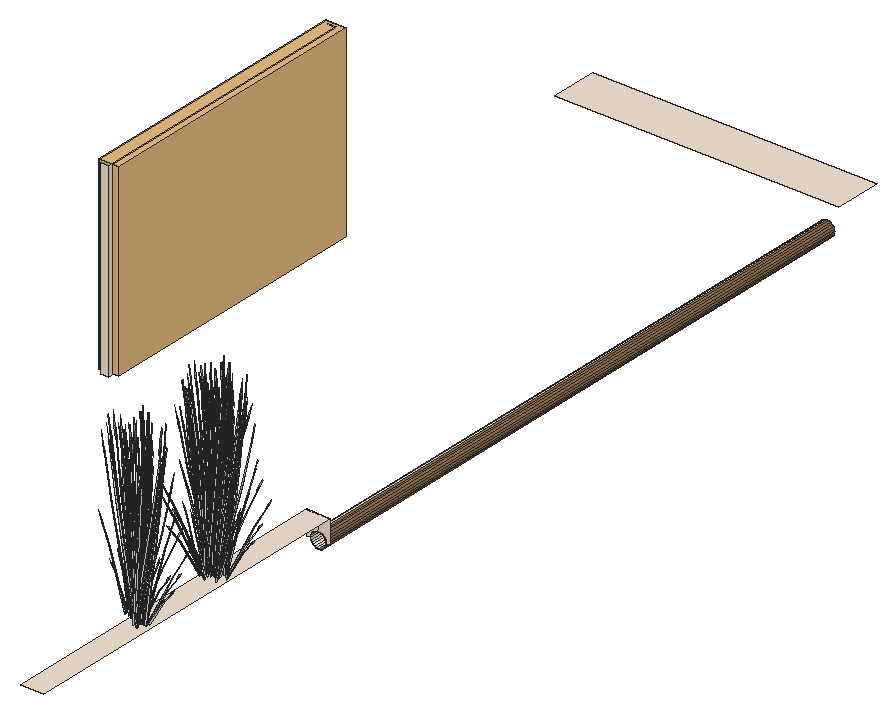
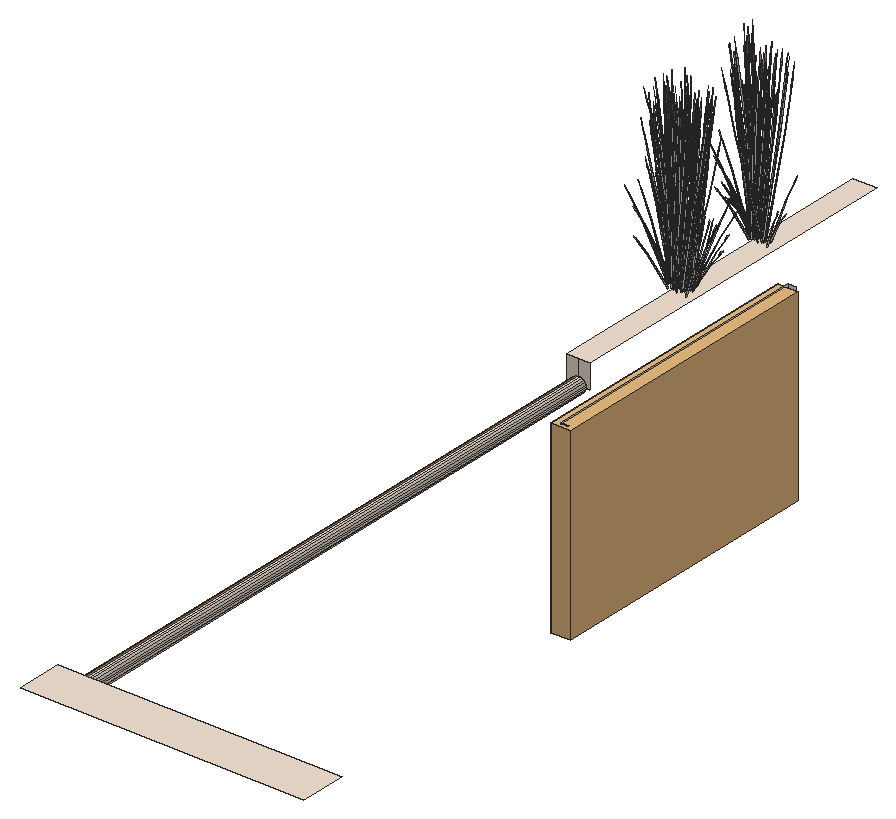
# SketchUp Ruby script. Lengths in inches.
U = 1.inch
M = Sketchup.active_model
def pt(a) = Geom::Point3d.new(a.map { |v| v * U })
def face(e, loops, mat)
  f = e.add_face(loops[0].map { |a| pt(a) })
  loops[1..].each { |l| e.add_face(l.map { |a| pt(a) }).erase! }
  f.material = f.back_material = mat if mat
  f
end
# faces: each face lists its corners as indices into pts; further lists are holes
def faces(e, pts, list, mat = nil) = list.each { |f| face(e, (f[0].is_a?(Array) ? f : [f]).map { |l| l.map { |i| pts[i] } }, mat) }
# xy, xz, yz: faces in a plane at the given z, y or x. An outline is a flat list of corners, or four numbers for a rectangle; further outlines are holes
def ring(l) = l.size == 4 ? [[l[0], l[1]], [l[2], l[1]], [l[2], l[3]], [l[0], l[3]]] : l.each_slice(2).to_a
def flat(e, list, mat, &to3) = list.each { |f| face(e, (f[0].is_a?(Array) ? f : [f]).map { |l| ring(l).map { |u, v| to3.(u, v) } }, mat) }
def xy(e, z, list, mat = nil) = flat(e, list, mat) { |x, y| [x, y, z] }
def xz(e, y, list, mat = nil) = flat(e, list, mat) { |x, z| [x, y, z] }
def yz(e, x, list, mat = nil) = flat(e, list, mat) { |y, z| [x, y, z] }
def lines(e, pts, list) = list.each { |a, b| e.add_line(pt(pts[a]), pt(pts[b])) }
# prism: a flat outline (further loops are holes) pulled along v
def prism(e, loops, v, mat = nil)
  f = face(e, loops, mat); d = Geom::Vector3d.new(v.map { |x| x * U })
  f.pushpull(f.normal.samedirection?(d) ? d.length : -d.length)
end
def box(e, o, s, mat = nil) = prism(e, [[o, [o[0] + s[0], o[1], o[2]], [o[0] + s[0], o[1] + s[1], o[2]], [o[0], o[1] + s[1], o[2]]]], [0, 0, s[2]], mat)
def at(x, y, z, deg = 0) = Geom::Transformation.translation(pt([x, y, z])) * Geom::Transformation.rotation(ORIGIN, Z_AXIS, deg.degrees)
def axes(o, x, y, z) = Geom::Transformation.new([*x, 0, *y, 0, *z, 0, *pt(o).to_a, 1])
def part(name) = M.definitions.add(name)
# library, detail: a bought-in or finely detailed component or shape, given as its bounding box
def library(name, o, s) = part(name).tap { |d| box(d.entities, o, s) }
def detail(e, o, s) = box(e.add_group.entities, o, s)
def put(e, d, t, mat = nil) = e.add_instance(d, t).tap { |i| i.material = mat if mat }
def group(e, t, mat = nil) = e.add_group.tap { |g| g.transformation = t; g.material = mat if mat }.entities
root = M.entities
M.materials.add("C01_Vanilla_Cream").color = [244, 228, 212]
M.materials.add("LightPink_Translucent").color = [144, 107, 117]
M.materials["LightPink_Translucent"].alpha = 0.75
M.materials.add("Wood_Floor_01_1K").color = [146, 111, 76]
c1 = part("blade")
p = [[2.15,0.21,22],[0,0.17,0],[0.09,0.45,0],[2.18,0.31,22],[2.29,0.31,22],[0.38,0.45,0],
  [2.48,0.24,33],[2.49,0.24,33],[2.48,0.22,33]]
faces(c1.entities,p,[[0,1,2,3],[4,5,2,3],[6,3,4,7],[8,0,3,6]])
c2 = part("seeds")
p = [[0.3,-0.1,1.38],[-0.01,-0.03,1.59],[-0.01,-0.03,0.03],[0.14,-0.07,-0.07],[0.29,-0.03,3],[0.15,0.01,3.11]]
faces(c2.entities,p,[[0,1,2,3],[1,0,4,5]],"LightPink_Translucent")
c3 = part("blade with seeds")
put(c3.entities,c1,at(0,0,0))
put(c3.entities,c2,axes([2.4,0.25,30.99],[1.5799,-0.05474,1.17369],[-0.12525,1.92788,0.29478],[-0.07173,-0.02425,1.56792]))
c4 = library("Double casement window",[0,0,0],[5.02,56.42,60])
xy(root,348,[[354,216,360,306.76],[288,324,290,396],[288,468,360,480]],"C01_Vanilla_Cream")
xz(root,306.76,[[354,342,354,348,357,348,357,344,356.48,343.93,356,343.73,355.59,343.41,355.27,343,355.07,342.52,355,342],[359,342,358.93,342.52,358.73,343,358.41,343.41,358,343.73,357.52,343.93,357,344,357,348,360,348,360,342]],"C01_Vanilla_Cream")
xz(root,324,[[288,348,290,396]],"C01_Vanilla_Cream")
xz(root,396,[[288,348,290,396]],"C01_Vanilla_Cream")
yz(root,290,[[[324,348,396,396],[327,351,358.5,393],[361.5,351,393,393]]],"C01_Vanilla_Cream")
p = [[357,306.76,340],[356.48,306.76,340.07],[356.48,468,340.07],[357,468,340],[357.52,306.76,340.07],[357.52,468,340.07],
  [356,306.76,340.27],[356,468,340.27],[358,306.76,340.27],[358,468,340.27],[355.59,306.76,340.59],[355.59,468,340.59],
  [358.41,306.76,340.59],[358.41,468,340.59],[355.27,306.76,341],[355.27,468,341],[358.73,306.76,341],[358.73,468,341],
  [355.07,306.76,341.48],[355.07,468,341.48],[358.93,306.76,341.48],[358.93,468,341.48],[355,306.76,342],[355,468,342],
  [359,306.76,342],[359,468,342],[355.07,306.76,342.52],[355.07,468,342.52],[358.93,306.76,342.52],[358.93,468,342.52],
  [355.27,306.76,343],[355.27,468,343],[358.73,306.76,343],[358.73,468,343],[355.59,306.76,343.41],[355.59,468,343.41],
  [358.41,306.76,343.41],[358.41,468,343.41],[356,306.76,343.73],[356,468,343.73],[358,306.76,343.73],[358,468,343.73],
  [356.48,306.76,343.93],[356.48,468,343.93],[357.52,306.76,343.93],[357.52,468,343.93],[357,306.76,344],[357,468,344]]
faces(root,p,[[0,1,2,3],[1,6,7,2],[6,10,11,7],[10,14,15,11],[14,18,19,15],[18,22,23,19],[22,26,27,23],[26,30,31,27],
  [30,34,35,31],[34,38,39,35],[38,42,43,39],[42,46,47,43]],"C01_Vanilla_Cream")
faces(root,p,[[4,0,3,5],[8,4,5,9],[12,8,9,13],[16,12,13,17],[20,16,17,21],[24,20,21,25],[28,24,25,29],[32,28,29,33],
  [36,32,33,37],[40,36,37,41],[44,40,41,45],[46,44,45,47]],"Wood_Floor_01_1K")
put(root,c3,axes([356.73,248.87,349.86],[0.59825,-0.13076,0.13232],[0.14773,0.48663,0.26315],[-0.05336,-0.0709,1.20305]))
put(root,c3,axes([357.96,247.03,350],[0.56211,-0.32708,-0.21822],[0.3738,0.46216,-0.37502],[0.13869,0.04694,1.19781]))
put(root,c3,axes([355.92,249.08,349.51],[-0.52105,-0.24633,-0.37238],[0.31144,-0.44171,0],[-0.11867,-0.0561,1.18128]))
put(root,c3,axes([359.38,246.16,349.51],[0.52105,0.24633,-0.37238],[-0.31144,0.44171,0],[0.11867,0.0561,1.18128]))
put(root,c3,axes([358.39,247.57,349.65],[0.62289,0,0],[0,0.51004,0],[0,0,1.33805]))
put(root,c3,axes([357.33,248.21,350],[-0.56211,0.32708,-0.21822],[-0.3738,-0.46216,-0.37502],[-0.13869,-0.04694,1.19781]))
put(root,c3,axes([358.57,246.37,349.86],[-0.59825,0.13076,0.13232],[-0.14773,-0.48663,0.26315],[0.05336,0.0709,1.20305]))
put(root,c3,axes([359.23,246.35,349.52],[0.13078,0.42928,-0.23233],[-0.51941,0.1219,0.23233],[0.10471,0.0495,1.0423]))
put(root,c3,axes([358.1875,247.31,349.79],[-0.70367,-0.1038,0.36899],[0.1432,-0.58624,0.1448],[0.10283,0.05661,1.2811]))
put(root,c3,axes([357.625,248.76,349.65],[-0.18165,-0.42474,0],[0.51872,-0.14874,0],[0,0,1.15778]))
put(root,c3,axes([357.28,248.35,349.96],[-0.1074,0.43968,0.1086],[-0.52474,-0.07632,-0.3101],[-0.0955,-0.04515,0.95058]))
put(root,c3,axes([358.31,248.7,349.64],[0.5845,-0.16716,-0.14398],[0.20539,0.48152,0.00006],[0.06452,-0.01848,1.30423]))
put(root,c3,axes([358.51,248.9,349.86],[0.16083,-0.48962,0.13232],[0.58854,0.13856,0.26315],[-0.10167,0.00238,1.20305]))
put(root,c3,axes([358.375,247.79,349.66],[0.38863,0.31822,0],[-0.38863,0.31822,0],[0,0,1.2695]))
put(root,c3,axes([359.43,247.65,349.86],[-0.43742,-0.35886,0.13232],[0.44081,-0.34807,0.26315],[-0.04831,0.07329,1.20305]))
put(root,c3,axes([358.62,247.11,349.54],[0.57914,0.08077,-0.46765],[-0.12221,0.49823,-0.12274],[0.17283,0.06037,1.03225]))
put(root,c3,axes([361.18,247.98,350.07],[-0.34399,0.08133,0.86145],[0.16192,-0.33614,0.63294],[0.18249,0.023,0.18974]))
put(root,c3,axes([357.5,248.95,349.65],[-0.56127,-0.22118,0],[0.27012,-0.45959,0],[0,0,1.2203]))
put(root,c3,axes([357.96,248.36,349.85],[-0.54364,-0.39653,-0.18894],[0.45745,-0.44527,0.41347],[-0.14639,0.04639,1.26162]))
put(root,c3,axes([356.53,249.12,349.86],[0.52105,0.24633,0.37238],[-0.31144,0.44171,0],[-0.11867,-0.0561,1.18128]))
put(root,c3,axes([358.37,247.42,350.04],[0.27012,-0.44393,0.33554],[0.56127,0.21365,-0.16149],[0,0.10233,1.07733]))
put(root,c3,axes([358.27,247.67,349.72],[0,0.56976,-0.04228],[-0.69617,0,0],[0,0.01791,1.34526]))
put(root,c3,axes([358.32,247.27,349.66],[0.33445,0.41351,-0.33554],[-0.50659,0.29119,0.16149],[0.10823,0.05117,1.07733]))
put(root,c3,axes([356.23,249.38,349.78],[-0.34808,0.49367,0],[-0.58235,-0.27531,-0.38706],[-0.13264,-0.0627,1.22783]))
put(root,c3,axes([359.79,247.66,349.86],[0,-0.49266,0.37238],[0.62289,0,0],[0,0.11221,1.18128]))
put(root,c3,axes([358.23,248.03,350.04],[0.60457,-0.03041,0.33554],[0.05467,0.50484,-0.16149],[-0.10823,0.05117,1.07733]))
put(root,c3,axes([358.6,247.52,349.96],[0.51872,-0.14368,0.1086],[0.18165,0.41027,-0.3101],[0,0.09029,0.95058]))
put(root,c3,axes([357.6875,248.28,349.66],[-0.60457,0.03041,-0.33554],[-0.05467,-0.50484,0.16149],[-0.10823,0.05117,1.07733]))
put(root,c3,axes([360.53,248.52,349.94],[-0.13408,-0.12117,1.07251],[0.17446,-0.40083,-0.23066],[0.27128,0.0543,0.45856]))
put(root,c3,axes([358.14,248.96,349.65],[0.56127,0.22118,0],[-0.27012,0.45959,0],[0,0,1.31215]))
put(root,c3,axes([358.36,249.45,349.64],[-0.34375,-0.4954,-0.03857],[0.58235,-0.27531,0.38706],[-0.1435,0.04717,1.22723]))
put(root,c3,axes([358.24,248.25,349.96],[0.41131,0.296,0.1086],[-0.34309,0.33395,-0.3101],[-0.0955,0.04515,0.95058]))
put(root,c3,axes([358.67,249.16,349.86],[0.52105,-0.24633,0.37238],[0.31144,0.44171,0],[-0.11867,0.0561,1.18128]))
put(root,c3,axes([357.93,248.77,349.72],[0.24206,0.56598,-0.04509],[-0.69162,0.19832,0],[0.00845,0.01976,1.2913]))
put(root,c3,axes([358.2,249.38,349.52],[-0.51941,-0.1219,-0.23233],[0.13078,-0.42928,0.23233],[-0.10471,0.0495,1.0423]))
put(root,c3,axes([354.45,248.51,349.94],[0.19348,0.04044,1.07251],[0.1247,0.41309,-0.23066],[-0.26282,0.07733,0.45856]))
put(root,c3,axes([360.21,247.75,349.78],[0.69617,0,0],[0,0.55062,-0.38706],[0,0.12541,1.22783]))
put(root,c3,axes([359.93,248.03,349.65],[-0.69582,-0.00394,-0.03732],[0,-0.55062,0.37457],[-0.02187,0.12535,1.18764]))
put(root,c3,axes([358.43,247.55,350],[0.62699,0.23507,-0.21822],[-0.3019,0.49615,-0.37502],[0.0197,0.12182,1.19781]))
put(root,c3,axes([354.05,249.38,350.07],[0.23202,-0.22328,0.86145],[0.09155,0.35348,0.63294],[-0.16768,0.06329,0.18974]))
put(root,c3,axes([359.79,248.11,349.52],[-0.38863,0.30738,-0.23233],[-0.38863,-0.30738,0.23233],[0,0.09901,1.0423]))
put(root,c3,axes([358.11,248.14,350],[0.06488,0.56215,-0.21822],[-0.6757,0.03399,-0.37502],[-0.11898,0.07488,1.19781]))
put(root,c3,axes([358.36,247.92,349.66],[-0.27012,0.44393,-0.33554],[-0.56127,-0.21365,0.16149],[0,0.10233,1.07733]))
put(root,c3,axes([357.71,248.57,349.54],[-0.375,0.3703,-0.46765],[-0.46584,-0.33578,-0.12274],[-0.15027,0.09237,1.03225]))
put(root,c3,axes([358.375,249.19,349.75],[0.697,0.16013,0.23067],[-0.17437,0.57237,-0.27369],[-0.11536,0.07164,1.23664]))
put(root,c3,axes([358.32,249.58,349.51],[-0.52105,0.24633,-0.37238],[-0.31144,-0.44171,0],[-0.11867,0.0561,1.18128]))
put(root,c3,axes([360.06,248.12,349.51],[0,0.49266,-0.37238],[-0.62289,0,0],[0,0.11221,1.18128]))
put(root,c3,axes([359.26,249.14,350.07],[-0.31347,-0.14166,0.86145],[0.40476,-0.14393,0.63294],[0.10917,0.12192,0.18974]))
put(root,c3,axes([358.8,249.5,349.78],[0.34808,0.49367,0],[-0.58235,0.27531,-0.38706],[-0.13264,0.0627,1.22783]))
put(root,c3,axes([359.35,249.67,349.12],[0.04056,-0.07113,1.32257],[0.51066,-0.20948,-0.20205],[0.15482,0.10842,0.22528]))
put(root,c3,axes([358.68,248.05,349.57],[0.20414,0.45107,-0.51909],[-0.58805,0.16245,-0.13624],[0.02256,0.15274,1.1458]))
put(root,c3,axes([354.66,249.61,349.12],[0.07468,0.04922,1.32257],[0.12663,0.45605,-0.20205],[-0.16551,0.09725,0.22528]))
put(root,c3,axes([359.3125,249.79,350],[-0.35702,-0.01545,0.78795],[0.23577,-0.32816,0.43504],[0.14104,0.11659,0.61808]))
put(root,c3,axes([358.15,248.99,349.94],[0.00982,-0.16331,1.07251],[0.4695,-0.18242,-0.23066],[0.14493,0.19547,0.45856]))
put(root,c3,axes([356.97,249.65,349.12],[0.0901,-0.02681,1.32257],[0.54199,0.14755,-0.20205],[0.01585,0.1663,0.22528]))
put(root,c3,axes([355.72,249.72,350.12],[0.50577,-0.08724,0.04881],[0.11627,0.35148,-0.64728],[-0.03206,0.17792,0.5802]))
put(root,c3,axes([355.6,250.09,349.94],[0.17569,-0.07772,1.07251],[0.43377,0.23434,-0.23066],[-0.12911,0.20277,0.45856]))
put(root,c3,axes([358.54,270.98,349.94],[-0.15825,0.09972,1.07251],[-0.47395,-0.17454,-0.23066],[0.08785,-0.21706,0.45856]))
put(root,c3,axes([356.09,270.79,349.94],[-0.03371,0.16116,1.07251],[-0.49286,0.13491,-0.23066],[-0.11521,-0.20831,0.45856]))
put(root,c3,axes([357.36,270.44,349.12],[-0.09338,0.01775,1.32257],[-0.51641,-0.1998,-0.20205],[0.00867,-0.16666,0.22528]))
put(root,c3,axes([355.6875,271.05,349.12],[-0.05393,0.0649,1.32257],[-0.545,0.13993,-0.20205],[-0.13166,-0.12729,0.22528]))
put(root,c3,axes([356.59,272.83,349.57],[-0.22864,-0.5052,-0.52377],[0.65862,-0.18195,-0.13747],[-0.02527,-0.17107,1.15612]))
put(root,c3,axes([359.64,271.29,349.12],[-0.08333,-0.03881,1.32257],[-0.21404,-0.4336,-0.20205],[0.14439,-0.11767,0.22528]))
put(root,c3,axes([356.5,271.38,349.78],[-0.34808,-0.49367,0],[0.58235,-0.27531,-0.38706],[0.13264,-0.0627,1.22783]))
put(root,c3,axes([357.26,270.79,349.6],[-0.38473,0.28263,-0.02919],[-0.35252,-0.30954,-0.13237],[-0.02482,-0.08771,0.43661]))
put(root,c3,axes([355.24,272.76,349.51],[0,-0.49266,-0.37238],[0.62289,0,0],[0,-0.11221,1.18128]))
put(root,c3,axes([356.97,271.3,349.51],[0.52105,-0.24633,-0.37238],[0.31144,0.44171,0],[0.11867,-0.0561,1.18128]))
put(root,c3,axes([360.0625,272.16,349.94],[-0.19889,-0.01459,1.07251],[-0.20376,-0.39145,-0.23066],[0.24434,-0.11074,0.45856]))
put(root,c3,axes([357.59,272.32,349.54],[0.375,-0.3703,-0.46765],[0.46584,0.33578,-0.12274],[0.15027,-0.09237,1.03225]))
put(root,c3,axes([356.93,272.96,349.66],[0.27012,-0.44393,-0.33554],[0.56127,0.21365,0.16149],[0,-0.10233,1.07733]))
put(root,c3,axes([357.18,272.74,350],[-0.06488,-0.56215,-0.21822],[0.6757,-0.03399,-0.37502],[0.11898,-0.07488,1.19781]))
put(root,c3,axes([355.51,272.77,349.52],[0.38863,-0.30738,-0.23233],[0.38863,0.30738,0.23233],[0,-0.09901,1.0423]))
put(root,c3,axes([355.35,271.3,349.6],[-0.1606,0.40228,-0.02919],[-0.4943,-0.12375,-0.13237],[-0.07505,-0.0658,0.43661]))
put(root,c3,axes([356.87,273.33,350],[-0.62699,-0.23507,-0.21822],[0.3019,-0.49615,-0.37502],[-0.0197,-0.12182,1.19781]))
put(root,c3,axes([355.08,273.14,349.78],[-0.69617,0,0],[0,-0.55062,-0.38706],[0,-0.12541,1.22783]))
put(root,c3,axes([355.2,272.15,349.94],[0.1087,0.13716,1.07251],[-0.25048,0.37284,-0.23066],[-0.25719,-0.08912,0.45856]))
put(root,c3,axes([357.09,271.5,349.52],[0.51941,0.1219,-0.23233],[-0.13078,0.42928,0.23233],[0.10471,-0.0495,1.0423]))
put(root,c3,axes([355.625,272.99,349.75],[-0.51786,0.4142,0.23067],[-0.51817,-0.40984,-0.27369],[-0.01808,-0.11762,1.23664]))
put(root,c3,axes([357.27,273.18,349.82],[0.6273,0.23878,0.18048],[-0.3019,0.49615,0.37502],[0,-0.11437,1.20407]))
put(root,c3,axes([357.03,273.86,349.83],[0.14756,-0.58378,-0.17572],[0.69966,0.10176,0.38453],[-0.12225,-0.08062,1.1733]))
put(root,c3,axes([357.07,272.85,350.04],[-0.60457,0.03041,0.33554],[-0.05467,-0.50484,-0.16149],[0.10823,-0.05117,1.07733]))
put(root,c3,axes([355.51,273.22,349.86],[0,0.49266,0.37238],[-0.62289,0,0],[0,-0.11221,1.18128]))
put(root,c3,axes([359.0625,271.51,349.78],[0.34808,-0.49367,0],[0.58235,0.27531,-0.38706],[0.13264,0.0627,1.22783]))
put(root,c3,axes([356.98,273.62,349.66],[-0.33445,-0.41351,-0.33554],[0.50659,-0.29119,0.16149],[-0.10823,-0.05117,1.07733]))
put(root,c3,axes([357.05,273.03,349.77],[0.24206,0.5509,0.34316],[-0.69162,0.19157,0.13466],[0.00845,-0.10123,1.19142]))
put(root,c3,axes([360.43,273.46,349.49],[-0.35858,0.05912,1.06187],[-0.05708,-0.47061,0.06078],[0.25115,-0.07123,0.60425]))
put(root,c3,axes([361.08,273.04,349.7],[-0.34516,-0.31503,-0.04866],[0.37803,-0.28865,-0.22062],[0.10711,-0.02032,0.72768]))
put(root,c3,axes([356.92,273.47,350.04],[-0.27012,0.44393,0.33554],[-0.56127,-0.21365,-0.16149],[0,-0.10233,1.07733]))
put(root,c3,axes([357.92,273.08,349.65],[0,-0.57005,0],[0.69617,0,0],[0,0,1.34592]))
put(root,c3,axes([358.76,271.76,349.86],[-0.52105,-0.24633,0.37238],[0.31144,-0.44171,0],[0.11867,0.0561,1.18128]))
put(root,c3,axes([356.68,273.78,349.54],[-0.57914,-0.08077,-0.46765],[0.12221,-0.49823,-0.12274],[-0.17283,-0.06037,1.03225]))
put(root,c3,axes([357.59,272.72,349.77],[-0.46162,0.4471,0.34316],[-0.54842,-0.39467,0.13466],[0.11129,-0.04462,1.19142]))
put(root,c3,axes([358.09,273.52,349.72],[-0.51786,-0.42404,-0.04598],[0.51817,-0.4243,0],[-0.01808,-0.01481,1.31678]))
put(root,c3,axes([356.79,271.99,349.86],[-0.16083,0.48962,0.13232],[-0.58854,-0.13856,0.26315],[0.10167,-0.00238,1.20305]))
put(root,c3,axes([356.54,272.38,349.2],[-0.548,0.19724,0.96696],[-0.17442,-0.56594,0.37572],[0.3365,0.00941,1.09981]))
put(root,c3,axes([358.01,272.53,349.96],[0.1074,-0.43968,0.1086],[0.52474,0.07632,-0.3101],[0.0955,0.04515,0.95058]))
put(root,c3,axes([357.11,273.57,349.77],[0.70367,0.1038,0.34316],[-0.1432,0.58624,0.13466],[-0.10283,-0.05661,1.19142]))
put(root,c3,axes([360.82,273.15,349.12],[-0.0291,-0.0748,1.32257],[0.20181,-0.43752,-0.20205],[0.20357,-0.00629,0.22528]))
put(root,c3,axes([354.81,273.07,349.12],[0.01412,0.07764,1.32257],[-0.28464,0.40547,-0.20205],[-0.20218,-0.02044,0.22528]))
put(root,c3,axes([357.79,272.65,350.04],[-0.33445,-0.41351,0.33554],[0.50659,-0.29119,-0.16149],[0.10823,0.05117,1.07733]))
put(root,c3,axes([356.0625,274.54,349.52],[-0.13078,-0.42928,-0.23233],[0.51941,-0.1219,0.23233],[-0.10471,-0.0495,1.0423]))
put(root,c3,axes([356.73,274.51,349.86],[0.59825,-0.13076,0.13232],[0.14773,0.48663,0.26315],[-0.05336,-0.0709,1.20305]))
put(root,c3,axes([357.96,272.67,350],[0.56211,-0.32708,-0.21822],[0.3738,0.46216,-0.37502],[0.13869,0.04694,1.19781]))
put(root,c3,axes([355.92,274.72,349.51],[-0.52105,-0.24633,-0.37238],[0.31144,-0.44171,0],[-0.11867,-0.0561,1.18128]))
put(root,c3,axes([359.38,271.8,349.51],[0.52105,0.24633,-0.37238],[-0.31144,0.44171,0],[0.11867,0.0561,1.18128]))
put(root,c3,axes([358.39,273.21,349.65],[0.62289,0,0],[0,0.51004,0],[0,0,1.33805]))
put(root,c3,axes([357.33,273.85,350],[-0.56211,0.32708,-0.21822],[-0.3738,-0.46216,-0.37502],[-0.13869,-0.04694,1.19781]))
put(root,c3,axes([358.57,272.01,349.86],[-0.59825,0.13076,0.13232],[-0.14773,-0.48663,0.26315],[0.05336,0.0709,1.20305]))
put(root,c3,axes([359.23,271.99,349.52],[0.13078,0.42928,-0.23233],[-0.51941,0.1219,0.23233],[0.10471,0.0495,1.0423]))
put(root,c3,axes([358.1875,272.95,349.79],[-0.70367,-0.1038,0.36899],[0.1432,-0.58624,0.1448],[0.10283,0.05661,1.2811]))
put(root,c3,axes([357.625,274.4,349.65],[-0.18165,-0.42474,0],[0.51872,-0.14874,0],[0,0,1.15778]))
put(root,c3,axes([357.28,273.99,349.96],[-0.1074,0.43968,0.1086],[-0.52474,-0.07632,-0.3101],[-0.0955,-0.04515,0.95058]))
put(root,c3,axes([358.31,274.34,349.64],[0.5845,-0.16716,-0.14398],[0.20539,0.48152,0.00006],[0.06452,-0.01848,1.30423]))
put(root,c3,axes([358.51,274.54,349.86],[0.16083,-0.48962,0.13232],[0.58854,0.13856,0.26315],[-0.10167,0.00238,1.20305]))
put(root,c3,axes([358.375,273.43,349.66],[0.38863,0.31822,0],[-0.38863,0.31822,0],[0,0,1.2695]))
put(root,c3,axes([359.43,273.29,349.86],[-0.43742,-0.35886,0.13232],[0.44081,-0.34807,0.26315],[-0.04831,0.07329,1.20305]))
put(root,c3,axes([358.62,272.75,349.54],[0.57914,0.08077,-0.46765],[-0.12221,0.49823,-0.12274],[0.17283,0.06037,1.03225]))
put(root,c3,axes([357.5,274.59,349.65],[-0.56127,-0.22118,0],[0.27012,-0.45959,0],[0,0,1.2203]))
put(root,c3,axes([357.96,274,349.85],[-0.54364,-0.39653,-0.18894],[0.45745,-0.44527,0.41347],[-0.14639,0.04639,1.26162]))
put(root,c3,axes([356.53,274.76,349.86],[0.52105,0.24633,0.37238],[-0.31144,0.44171,0],[-0.11867,-0.0561,1.18128]))
put(root,c3,axes([358.37,273.05,350.04],[0.27012,-0.44393,0.33554],[0.56127,0.21365,-0.16149],[0,0.10233,1.07733]))
put(root,c3,axes([358.27,273.31,349.72],[0,0.56976,-0.04228],[-0.69617,0,0],[0,0.01791,1.34526]))
put(root,c3,axes([358.32,272.9,349.66],[0.33445,0.41351,-0.33554],[-0.50659,0.29119,0.16149],[0.10823,0.05117,1.07733]))
put(root,c3,axes([356.23,275.02,349.78],[-0.34808,0.49367,0],[-0.58235,-0.27531,-0.38706],[-0.13264,-0.0627,1.22783]))
put(root,c3,axes([359.79,273.3,349.86],[0,-0.49266,0.37238],[0.62289,0,0],[0,0.11221,1.18128]))
put(root,c3,axes([358.23,273.67,350.04],[0.60457,-0.03041,0.33554],[0.05467,0.50484,-0.16149],[-0.10823,0.05117,1.07733]))
put(root,c3,axes([358.6,273.16,349.96],[0.51872,-0.14368,0.1086],[0.18165,0.41027,-0.3101],[0,0.09029,0.95058]))
put(root,c3,axes([357.6875,273.91,349.66],[-0.60457,0.03041,-0.33554],[-0.05467,-0.50484,0.16149],[-0.10823,0.05117,1.07733]))
put(root,c3,axes([360.53,274.16,349.94],[-0.13408,-0.12117,1.07251],[0.17446,-0.40083,-0.23066],[0.27128,0.0543,0.45856]))
put(root,c3,axes([358.14,274.6,349.65],[0.56127,0.22118,0],[-0.27012,0.45959,0],[0,0,1.31215]))
put(root,c3,axes([358.36,275.09,349.64],[-0.34375,-0.4954,-0.03857],[0.58235,-0.27531,0.38706],[-0.1435,0.04717,1.22723]))
put(root,c3,axes([358.24,273.89,349.96],[0.41131,0.296,0.1086],[-0.34309,0.33395,-0.3101],[-0.0955,0.04515,0.95058]))
put(root,c3,axes([358.67,274.8,349.86],[0.52105,-0.24633,0.37238],[0.31144,0.44171,0],[-0.11867,0.0561,1.18128]))
put(root,c3,axes([357.93,274.41,349.72],[0.24206,0.56598,-0.04509],[-0.69162,0.19832,0],[0.00845,0.01976,1.2913]))
put(root,c3,axes([358.2,275.02,349.52],[-0.51941,-0.1219,-0.23233],[0.13078,-0.42928,0.23233],[-0.10471,0.0495,1.0423]))
put(root,c3,axes([354.45,274.15,349.94],[0.19348,0.04044,1.07251],[0.1247,0.41309,-0.23066],[-0.26282,0.07733,0.45856]))
put(root,c3,axes([360.21,273.39,349.78],[0.69617,0,0],[0,0.55062,-0.38706],[0,0.12541,1.22783]))
put(root,c3,axes([359.93,273.67,349.65],[-0.69582,-0.00394,-0.03732],[0,-0.55062,0.37457],[-0.02187,0.12535,1.18764]))
put(root,c3,axes([358.43,273.1875,350],[0.62699,0.23507,-0.21822],[-0.3019,0.49615,-0.37502],[0.0197,0.12182,1.19781]))
put(root,c3,axes([359.79,273.75,349.52],[-0.38863,0.30738,-0.23233],[-0.38863,-0.30738,0.23233],[0,0.09901,1.0423]))
put(root,c3,axes([358.11,273.78,350],[0.06488,0.56215,-0.21822],[-0.6757,0.03399,-0.37502],[-0.11898,0.07488,1.19781]))
put(root,c3,axes([358.36,273.56,349.66],[-0.27012,0.44393,-0.33554],[-0.56127,-0.21365,0.16149],[0,0.10233,1.07733]))
put(root,c3,axes([357.71,274.21,349.54],[-0.375,0.3703,-0.46765],[-0.46584,-0.33578,-0.12274],[-0.15027,0.09237,1.03225]))
put(root,c3,axes([358.375,274.83,349.75],[0.697,0.16013,0.23067],[-0.17437,0.57237,-0.27369],[-0.11536,0.07164,1.23664]))
put(root,c3,axes([358.32,275.22,349.51],[-0.52105,0.24633,-0.37238],[-0.31144,-0.44171,0],[-0.11867,0.0561,1.18128]))
put(root,c3,axes([360.06,273.76,349.51],[0,0.49266,-0.37238],[-0.62289,0,0],[0,0.11221,1.18128]))
put(root,c3,axes([358.8,275.14,349.78],[0.34808,0.49367,0],[-0.58235,0.27531,-0.38706],[-0.13264,0.0627,1.22783]))
put(root,c3,axes([359.35,275.31,349.12],[0.04056,-0.07113,1.32257],[0.51066,-0.20948,-0.20205],[0.15482,0.10842,0.22528]))
put(root,c3,axes([358.68,273.69,349.57],[0.20414,0.45107,-0.51909],[-0.58805,0.16245,-0.13624],[0.02256,0.15274,1.1458]))
put(root,c3,axes([354.66,275.25,349.12],[0.07468,0.04922,1.32257],[0.12663,0.45605,-0.20205],[-0.16551,0.09725,0.22528]))
put(root,c3,axes([359.3125,275.43,350],[-0.35702,-0.01545,0.78795],[0.23577,-0.32816,0.43504],[0.14104,0.11659,0.61808]))
put(root,c3,axes([358.15,274.63,349.94],[0.00982,-0.16331,1.07251],[0.4695,-0.18242,-0.23066],[0.14493,0.19547,0.45856]))
put(root,c3,axes([356.97,275.29,349.12],[0.0901,-0.02681,1.32257],[0.54199,0.14755,-0.20205],[0.01585,0.1663,0.22528]))
put(root,c3,axes([355.72,275.36,350.12],[0.50577,-0.08724,0.04881],[0.11627,0.35148,-0.64728],[-0.03206,0.17792,0.5802]))
put(root,c3,axes([355.6,275.73,349.94],[0.17569,-0.07772,1.07251],[0.43377,0.23434,-0.23066],[-0.12911,0.20277,0.45856]))
put(root,c4,axes([286.7,325.0625,348.3],[1,0,0],[0,1.27666,0],[0,0,0.79394]))
